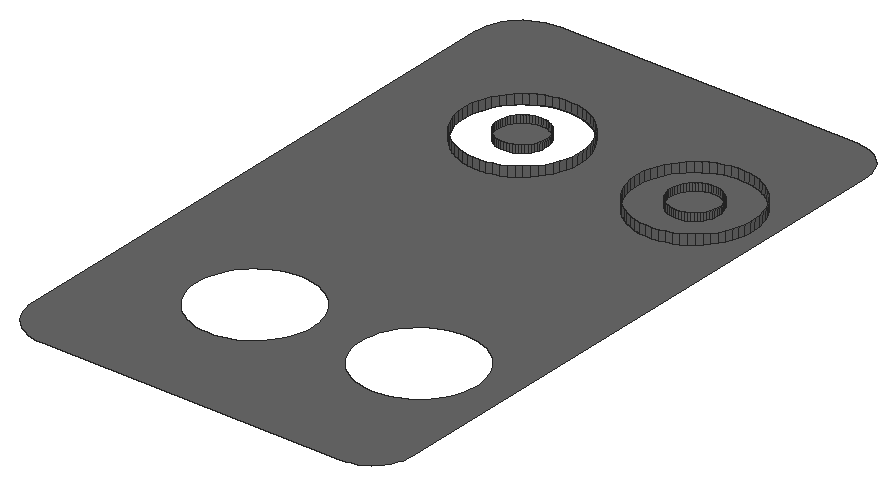
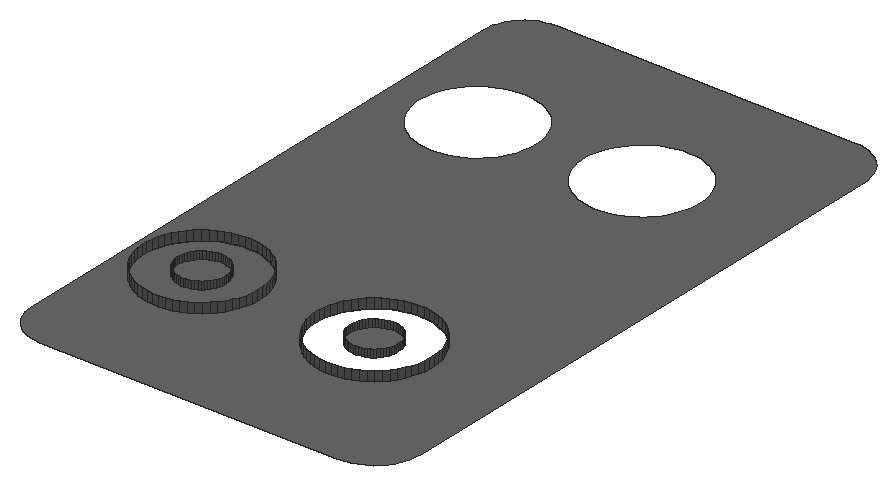
# SketchUp Ruby script. Lengths in inches.
U = 1.inch
M = Sketchup.active_model
def pt(a) = Geom::Point3d.new(a.map { |v| v * U })
def face(e, loops, mat)
  f = e.add_face(loops[0].map { |a| pt(a) })
  loops[1..].each { |l| e.add_face(l.map { |a| pt(a) }).erase! }
  f.material = f.back_material = mat if mat
  f
end
# faces: each face lists its corners as indices into pts; further lists are holes
def faces(e, pts, list, mat = nil) = list.each { |f| face(e, (f[0].is_a?(Array) ? f : [f]).map { |l| l.map { |i| pts[i] } }, mat) }
# xy, xz, yz: faces in a plane at the given z, y or x. An outline is a flat list of corners, or four numbers for a rectangle; further outlines are holes
def ring(l) = l.size == 4 ? [[l[0], l[1]], [l[2], l[1]], [l[2], l[3]], [l[0], l[3]]] : l.each_slice(2).to_a
def flat(e, list, mat, &to3) = list.each { |f| face(e, (f[0].is_a?(Array) ? f : [f]).map { |l| ring(l).map { |u, v| to3.(u, v) } }, mat) }
def xy(e, z, list, mat = nil) = flat(e, list, mat) { |x, y| [x, y, z] }
def xz(e, y, list, mat = nil) = flat(e, list, mat) { |x, z| [x, y, z] }
def yz(e, x, list, mat = nil) = flat(e, list, mat) { |y, z| [x, y, z] }
def lines(e, pts, list) = list.each { |a, b| e.add_line(pt(pts[a]), pt(pts[b])) }
# prism: a flat outline (further loops are holes) pulled along v
def prism(e, loops, v, mat = nil)
  f = face(e, loops, mat); d = Geom::Vector3d.new(v.map { |x| x * U })
  f.pushpull(f.normal.samedirection?(d) ? d.length : -d.length)
end
def box(e, o, s, mat = nil) = prism(e, [[o, [o[0] + s[0], o[1], o[2]], [o[0] + s[0], o[1] + s[1], o[2]], [o[0], o[1] + s[1], o[2]]]], [0, 0, s[2]], mat)
def at(x, y, z, deg = 0) = Geom::Transformation.translation(pt([x, y, z])) * Geom::Transformation.rotation(ORIGIN, Z_AXIS, deg.degrees)
def axes(o, x, y, z) = Geom::Transformation.new([*x, 0, *y, 0, *z, 0, *pt(o).to_a, 1])
def part(name) = M.definitions.add(name)
# library, detail: a bought-in or finely detailed component or shape, given as its bounding box
def library(name, o, s) = part(name).tap { |d| box(d.entities, o, s) }
def detail(e, o, s) = box(e.add_group.entities, o, s)
def put(e, d, t, mat = nil) = e.add_instance(d, t).tap { |i| i.material = mat if mat }
def group(e, t, mat = nil) = e.add_group.tap { |g| g.transformation = t; g.material = mat if mat }.entities
root = M.entities
M.materials.add("[0134_DimGray]").color = [105, 105, 105]
xy(root,118,[[[56.8,138.66,118.35,138.66,119.44,138.73,120.52,138.94,121.55,139.3,122.54,139.78,123.45,140.39,124.27,141.11,124.99,141.9375,125.6,142.85,126.09,143.83,126.44,144.87,126.65,145.94,126.73,147.04,126.73,263.91,126.65,265,126.44,266.08,126.09,267.11,125.6,268.1,124.99,269.01,124.27,269.83,123.45,270.55,122.54,271.16,121.55,271.65,120.52,272,119.44,272.21,118.35,272.28,56.8,272.28,55.54,272.2,54.3,271.96,53.11,271.55,51.98,270.99,50.93,270.29,49.98,269.46,49.15,268.51,48.45,267.47,47.9,266.34,47.49,265.14,47.25,263.91,47.16,262.65,47.16,148.29,47.25,147.04,47.49,145.8,47.9,144.61,48.45,143.48,49.15,142.43,49.98,141.48,50.93,140.65,51.98,139.95,53.11,139.39,54.3,138.99,55.54,138.74],[75.05,157.99,73.8,158.11,72.57,158.36,71.375,158.74,70.22,159.25,69.13,159.87,68.11,160.6,67.17,161.43,66.33,162.36,65.58,163.37,64.94,164.46,64.43,165.6,64.03,166.79,63.76,168.02,63.62,169.27,63.61,170.52,63.74,171.77,63.99,173,64.37,174.2,64.87,175.35,65.49,176.44,66.22,177.46,67.06,178.4,67.99,179.25,69,179.99,70.08,180.63,71.23,181.15,72.42,181.54,73.64,181.8125,74.89,181.95,76.15,181.96,77.4,181.84,78.63,181.59,79.83,181.21,80.98,180.7,82.07,180.08,83.09,179.35,84.03,178.52,84.875,177.59,85.62,176.58,86.26,175.49,86.77,174.35,87.17,173.16,87.44,171.93,87.58,170.68,87.59,169.43,87.46,168.18,87.21,166.95,86.83,165.75,86.33,164.6,85.71,163.51,84.98,162.48,84.14,161.55,83.21,160.7,82.2,159.95,81.12,159.32,79.98,158.8,78.78,158.4,77.56,158.13,76.31,158],[75.05,227.2,73.8,227.32,72.57,227.58,71.375,227.96,70.22,228.46,69.13,229.08,68.11,229.8125,67.17,230.65,66.33,231.57,65.58,232.58,64.94,233.67,64.43,234.8125,64.03,236,63.76,237.23,63.62,238.48,63.61,239.74,63.74,240.99,63.99,242.22,64.37,243.41,64.87,244.5625,65.49,245.66,66.22,246.68,67.06,247.62,67.99,248.46,69,249.21,70.08,249.84,71.23,250.36,72.42,250.76,73.64,251.03,74.89,251.17,76.15,251.18,77.4,251.05,78.63,250.8,79.83,250.42,80.98,249.92,82.07,249.3,83.09,248.5625,84.03,247.73,84.875,246.8,85.62,245.79,86.26,244.71,86.77,243.5625,87.17,242.37,87.44,241.14,87.58,239.9,87.59,238.64,87.46,237.39,87.21,236.16,86.83,234.96,86.33,233.8125,85.71,232.72,84.98,231.7,84.14,230.76,83.21,229.91,82.2,229.17,81.12,228.53,79.98,228.01,78.78,227.62,77.56,227.35,76.31,227.21],[107.89,159.41,106.64,159.53,105.41,159.78,104.21,160.16,103.0625,160.67,101.97,161.29,100.95,162.02,100.01,162.85,99.16,163.78,98.42,164.79,97.78,165.875,97.26,167.02,96.87,168.21,96.6,169.4375,96.46,170.6875,96.45,171.94,96.57,173.19,96.83,174.42,97.21,175.62,97.71,176.77,98.33,177.86,99.0625,178.88,99.9,179.82,100.82,180.67,101.84,181.42,102.92,182.05,104.0625,182.57,105.26,182.97,106.48,183.23,107.73,183.375,108.99,183.38,110.24,183.26,111.47,183.01,112.66,182.625,113.81,182.125,114.91,181.5,115.93,180.77,116.87,179.9375,117.71,179.01,118.46,178,119.09,176.91,119.61,175.77,120.01,174.58,120.28,173.35,120.42,172.1,120.43,170.85,120.3,169.6,120.05,168.37,119.67,167.17,119.17,166.02,118.55,164.93,117.8125,163.91,116.98,162.97,116.05,162.12,115.04,161.375,113.96,160.74,112.8125,160.22,111.62,159.83,110.39,159.56,109.15,159.42],[110.81,227.1,109.56,227.22,108.33,227.47,107.13,227.85,105.98,228.36,104.89,228.98,103.86,229.71,102.93,230.54,102.08,231.47,101.33,232.48,100.7,233.57,100.18,234.71,99.78,235.9,99.51,237.13,99.375,238.38,99.37,239.63,99.49,240.88,99.74,242.11,100.12,243.3125,100.625,244.46,101.25,245.55,101.98,246.58,102.8125,247.51,103.74,248.36,104.75,249.11,105.83,249.74,106.98,250.26,108.17,250.66,109.4,250.93,110.65,251.07,111.9,251.07,113.15,250.95,114.38,250.7,115.58,250.32,116.73,249.81,117.82,249.19,118.84,248.46,119.78,247.63,120.63,246.7,121.375,245.6875,122.01,244.61,122.53,243.46,122.92,242.27,123.19,241.04,123.33,239.79,123.34,238.54,123.22,237.29,122.97,236.06,122.59,234.86,122.08,233.71,121.46,232.62,120.73,231.6,119.9,230.66,118.97,229.8125,117.96,229.07,116.875,228.43,115.73,227.91,114.54,227.52,113.31,227.25,112.0625,227.11]],[110.81,227.1,109.56,227.22,108.33,227.47,107.13,227.85,105.98,228.36,104.89,228.98,103.86,229.71,102.93,230.54,102.08,231.47,101.33,232.48,100.7,233.57,100.18,234.71,99.78,235.9,99.51,237.13,99.375,238.38,99.37,239.63,99.49,240.88,99.74,242.11,100.12,243.3125,100.625,244.46,101.25,245.55,101.98,246.58,102.8125,247.51,103.74,248.36,104.75,249.11,105.83,249.74,106.98,250.26,108.17,250.66,109.4,250.93,110.65,251.07,111.9,251.07,113.15,250.95,114.38,250.7,115.58,250.32,116.73,249.81,117.82,249.19,118.84,248.46,119.78,247.63,120.63,246.7,121.375,245.6875,122.01,244.61,122.53,243.46,122.92,242.27,123.19,241.04,123.33,239.79,123.34,238.54,123.22,237.29,122.97,236.06,122.59,234.86,122.08,233.71,121.46,232.62,120.73,231.6,119.9,230.66,118.97,229.8125,117.96,229.07,116.875,228.43,115.73,227.91,114.54,227.52,113.31,227.25,112.0625,227.11]],"[0134_DimGray]")
xy(root,118.5,[[111.53,234.09,112.05,234.14,112.5625,234.23,113.0625,234.39,113.55,234.59,114,234.85,114.43,235.15,114.83,235.49,115.18,235.87,115.5,236.29,115.77,236.74,115.99,237.21,116.16,237.71,116.28,238.22,116.34,238.74,116.35,239.26,116.31,239.78,116.21,240.3,116.05,240.8,115.85,241.28,115.59,241.74,115.29,242.16,114.95,242.56,114.57,242.92,114.15,243.23,113.7,243.5,113.23,243.72,112.73,243.89,112.22,244.01,111.7,244.07,111.18,244.08,110.66,244.04,110.14,243.9375,109.64,243.78,109.16,243.58,108.7,243.33,108.28,243.03,107.88,242.68,107.52,242.3,107.21,241.88,106.9375,241.43,106.72,240.96,106.55,240.46,106.43,239.95,106.37,239.44,106.36,238.91,106.4,238.39,106.5,237.875,106.66,237.375,106.86,236.89,107.11,236.4375,107.41,236.01,107.76,235.61,108.14,235.26,108.56,234.94,109.01,234.67,109.48,234.45,109.98,234.28,110.49,234.16,111.01,234.1],[75.77,234.19,76.3,234.24,76.81,234.34,77.31,234.49,77.79,234.69,78.25,234.95,78.68,235.25,79.07,235.59,79.43,235.97,79.75,236.39,80.01,236.84,80.24,237.31,80.41,237.81,80.52,238.32,80.59,238.84,80.6,239.36,80.55,239.88,80.45,240.4,80.3,240.9,80.09,241.38,79.84,241.84,79.54,242.27,79.2,242.66,78.8125,243.02,78.4,243.33,77.95,243.6,77.47,243.82,76.98,243.99,76.47,244.11,75.95,244.18,75.43,244.18,74.9,244.14,74.39,244.04,73.89,243.89,73.41,243.68,72.95,243.43,72.52,243.13,72.125,242.78,71.77,242.4,71.45,241.98,71.19,241.53,70.96,241.0625,70.79,240.57,70.68,240.06,70.61,239.54,70.6,239.01,70.65,238.49,70.75,237.98,70.9,237.48,71.11,237,71.36,236.54,71.66,236.11,72,235.71,72.39,235.36,72.8,235.04,73.25,234.77,73.73,234.55,74.22,234.38,74.73,234.26,75.25,234.2]],"[0134_DimGray]")
xz(root,244.18,[[75.43,118.5,75.95,120]],"[0134_DimGray]")
xz(root,251.07,[[110.65,118,111.9,120]],"[0134_DimGray]")
p = [[109.56,227.22,118],[110.81,227.1,118],[110.81,227.1,120],[109.56,227.22,120],[112.0625,227.11,118],[112.0625,227.11,120],
  [113.31,227.25,118],[113.31,227.25,120],[73.8,227.32,118],[75.05,227.2,118],[75.05,227.2,120],[73.8,227.32,120],
  [76.31,227.21,118],[76.31,227.21,120],[77.56,227.35,118],[77.56,227.35,120],[108.33,227.47,118],[108.33,227.47,120],
  [114.54,227.52,118],[114.54,227.52,120],[72.57,227.58,118],[72.57,227.58,120],[78.78,227.62,118],[78.78,227.62,120],
  [107.13,227.85,118],[107.13,227.85,120],[115.73,227.91,118],[115.73,227.91,120],[71.375,227.96,118],[71.375,227.96,120],
  [79.98,228.01,118],[79.98,228.01,120],[105.98,228.36,118],[105.98,228.36,120],[116.875,228.43,118],[116.875,228.43,120],
  [70.22,228.46,118],[70.22,228.46,120],[81.12,228.53,118],[81.12,228.53,120],[104.89,228.98,118],[104.89,228.98,120],
  [117.96,229.07,118],[117.96,229.07,120],[69.13,229.08,118],[69.13,229.08,120],[82.2,229.17,118],[82.2,229.17,120],
  [103.86,229.71,118],[103.86,229.71,120],[68.11,229.8125,118],[68.11,229.8125,120],[118.97,229.8125,118],[118.97,229.8125,120],
  [83.21,229.91,118],[83.21,229.91,120],[102.93,230.54,118],[102.93,230.54,120],[67.17,230.65,118],[67.17,230.65,120],
  [119.9,230.66,118],[119.9,230.66,120],[84.14,230.76,118],[84.14,230.76,120],[102.08,231.47,118],[102.08,231.47,120],
  [66.33,231.57,118],[66.33,231.57,120],[120.73,231.6,118],[120.73,231.6,120],[84.98,231.7,118],[84.98,231.7,120],
  [101.33,232.48,118],[101.33,232.48,120],[65.58,232.58,118],[65.58,232.58,120],[121.46,232.62,118],[121.46,232.62,120],
  [85.71,232.72,118],[85.71,232.72,120],[100.7,233.57,118],[100.7,233.57,120],[64.94,233.67,118],[64.94,233.67,120],
  [122.08,233.71,118],[122.08,233.71,120],[86.33,233.8125,118],[86.33,233.8125,120],[100.18,234.71,118],[100.18,234.71,120],
  [64.43,234.8125,118],[64.43,234.8125,120],[122.59,234.86,118],[122.59,234.86,120],[86.83,234.96,118],[86.83,234.96,120],
  [99.78,235.9,118],[99.78,235.9,120],[64.03,236,118],[64.03,236,120],[122.97,236.06,118],[122.97,236.06,120],
  [87.21,236.16,118],[87.21,236.16,120],[99.51,237.13,118],[99.51,237.13,120],[63.76,237.23,118],[63.76,237.23,120],
  [123.22,237.29,118],[123.22,237.29,120],[87.46,237.39,118],[87.46,237.39,120],[99.375,238.38,118],[99.375,238.38,120],
  [63.62,238.48,118],[63.62,238.48,120],[123.34,238.54,118],[123.34,238.54,120],[87.59,238.64,118],[87.59,238.64,120],
  [99.37,239.63,118],[99.37,239.63,120],[63.61,239.74,118],[63.61,239.74,120],[123.33,239.79,118],[123.33,239.79,120],
  [87.58,239.9,118],[87.58,239.9,120],[99.49,240.88,118],[99.49,240.88,120],[63.74,240.99,118],[63.74,240.99,120],
  [123.19,241.04,118],[123.19,241.04,120],[87.44,241.14,118],[87.44,241.14,120],[99.74,242.11,118],[99.74,242.11,120],
  [63.99,242.22,118],[63.99,242.22,120],[122.92,242.27,118],[122.92,242.27,120],[87.17,242.37,118],[87.17,242.37,120],
  [100.12,243.3125,118],[100.12,243.3125,120],[64.37,243.41,118],[64.37,243.41,120],[122.53,243.46,118],[122.53,243.46,120],
  [86.77,243.5625,118],[86.77,243.5625,120],[100.625,244.46,118],[100.625,244.46,120],[64.87,244.5625,118],[64.87,244.5625,120],
  [122.01,244.61,118],[122.01,244.61,120],[86.26,244.71,118],[86.26,244.71,120],[101.25,245.55,118],[101.25,245.55,120],
  [65.49,245.66,118],[65.49,245.66,120],[121.375,245.6875,118],[121.375,245.6875,120],[85.62,245.79,118],[85.62,245.79,120],
  [101.98,246.58,118],[101.98,246.58,120],[66.22,246.68,118],[66.22,246.68,120],[120.63,246.7,118],[120.63,246.7,120],
  [84.875,246.8,118],[84.875,246.8,120],[102.8125,247.51,118],[102.8125,247.51,120],[67.06,247.62,118],[67.06,247.62,120],
  [119.78,247.63,118],[119.78,247.63,120],[84.03,247.73,118],[84.03,247.73,120],[103.74,248.36,118],[103.74,248.36,120],
  [67.99,248.46,118],[67.99,248.46,120],[118.84,248.46,118],[118.84,248.46,120],[83.09,248.5625,118],[83.09,248.5625,120],
  [104.75,249.11,118],[104.75,249.11,120],[69,249.21,118],[69,249.21,120],[117.82,249.19,118],[117.82,249.19,120],
  [82.07,249.3,118],[82.07,249.3,120],[105.83,249.74,118],[105.83,249.74,120],[70.08,249.84,118],[70.08,249.84,120],
  [116.73,249.81,118],[116.73,249.81,120],[80.98,249.92,118],[80.98,249.92,120],[106.98,250.26,118],[106.98,250.26,120],
  [71.23,250.36,118],[71.23,250.36,120],[115.58,250.32,118],[115.58,250.32,120],[79.83,250.42,118],[79.83,250.42,120],
  [108.17,250.66,118],[108.17,250.66,120],[114.38,250.7,118],[114.38,250.7,120],[72.42,250.76,118],[72.42,250.76,120],
  [78.63,250.8,118],[78.63,250.8,120],[109.4,250.93,118],[109.4,250.93,120],[113.15,250.95,118],[113.15,250.95,120],
  [73.64,251.03,118],[73.64,251.03,120],[77.4,251.05,118],[77.4,251.05,120],[110.65,251.07,118],[110.65,251.07,120],
  [74.89,251.17,118],[74.89,251.17,120],[111.9,251.07,118],[111.9,251.07,120],[76.15,251.18,118],[76.15,251.18,120],
  [110.49,234.16,120],[111.01,234.1,120],[111.01,234.1,118.5],[110.49,234.16,118.5],[111.53,234.09,120],[111.53,234.09,118.5],
  [112.05,234.14,120],[112.05,234.14,118.5],[112.5625,234.23,120],[112.5625,234.23,118.5],[74.73,234.26,120],[75.25,234.2,120],
  [75.25,234.2,118.5],[74.73,234.26,118.5],[75.77,234.19,120],[75.77,234.19,118.5],[76.3,234.24,120],[76.3,234.24,118.5],
  [76.81,234.34,120],[76.81,234.34,118.5],[109.98,234.28,120],[109.98,234.28,118.5],[113.0625,234.39,120],[113.0625,234.39,118.5],
  [74.22,234.38,120],[74.22,234.38,118.5],[77.31,234.49,120],[77.31,234.49,118.5],[109.48,234.45,120],[109.48,234.45,118.5],
  [73.73,234.55,120],[73.73,234.55,118.5],[113.55,234.59,120],[113.55,234.59,118.5],[77.79,234.69,120],[77.79,234.69,118.5],
  [109.01,234.67,120],[109.01,234.67,118.5],[73.25,234.77,120],[73.25,234.77,118.5],[114,234.85,120],[114,234.85,118.5],
  [78.25,234.95,120],[78.25,234.95,118.5],[108.56,234.94,120],[108.56,234.94,118.5],[72.8,235.04,120],[72.8,235.04,118.5],
  [114.43,235.15,120],[114.43,235.15,118.5],[78.68,235.25,120],[78.68,235.25,118.5],[108.14,235.26,120],[108.14,235.26,118.5],
  [72.39,235.36,120],[72.39,235.36,118.5],[114.83,235.49,120],[114.83,235.49,118.5],[79.07,235.59,120],[79.07,235.59,118.5],
  [107.76,235.61,120],[107.76,235.61,118.5],[72,235.71,120],[72,235.71,118.5],[115.18,235.87,120],[115.18,235.87,118.5],
  [79.43,235.97,120],[79.43,235.97,118.5],[107.41,236.01,120],[107.41,236.01,118.5],[71.66,236.11,120],[71.66,236.11,118.5],
  [115.5,236.29,120],[115.5,236.29,118.5],[79.75,236.39,120],[79.75,236.39,118.5],[107.11,236.4375,120],[107.11,236.4375,118.5],
  [71.36,236.54,120],[71.36,236.54,118.5],[115.77,236.74,120],[115.77,236.74,118.5],[80.01,236.84,120],[80.01,236.84,118.5],
  [106.86,236.89,120],[106.86,236.89,118.5],[71.11,237,120],[71.11,237,118.5],[115.99,237.21,120],[115.99,237.21,118.5],
  [80.24,237.31,120],[80.24,237.31,118.5],[106.66,237.375,120],[106.66,237.375,118.5],[70.9,237.48,120],[70.9,237.48,118.5],
  [116.16,237.71,120],[116.16,237.71,118.5],[80.41,237.81,120],[80.41,237.81,118.5],[106.5,237.875,120],[106.5,237.875,118.5],
  [70.75,237.98,120],[70.75,237.98,118.5],[116.28,238.22,120],[116.28,238.22,118.5],[80.52,238.32,120],[80.52,238.32,118.5],
  [106.4,238.39,120],[106.4,238.39,118.5],[70.65,238.49,120],[70.65,238.49,118.5],[116.34,238.74,120],[116.34,238.74,118.5],
  [80.59,238.84,120],[80.59,238.84,118.5],[106.36,238.91,120],[106.36,238.91,118.5],[70.6,239.01,120],[70.6,239.01,118.5],
  [116.35,239.26,120],[116.35,239.26,118.5],[80.6,239.36,120],[80.6,239.36,118.5],[106.37,239.44,120],[106.37,239.44,118.5],
  [70.61,239.54,120],[70.61,239.54,118.5],[116.31,239.78,120],[116.31,239.78,118.5],[80.55,239.88,120],[80.55,239.88,118.5],
  [106.43,239.95,120],[106.43,239.95,118.5],[70.68,240.06,120],[70.68,240.06,118.5],[116.21,240.3,120],[116.21,240.3,118.5],
  [80.45,240.4,120],[80.45,240.4,118.5],[106.55,240.46,120],[106.55,240.46,118.5],[70.79,240.57,120],[70.79,240.57,118.5],
  [116.05,240.8,120],[116.05,240.8,118.5],[80.3,240.9,120],[80.3,240.9,118.5],[106.72,240.96,120],[106.72,240.96,118.5],
  [70.96,241.0625,120],[70.96,241.0625,118.5],[115.85,241.28,120],[115.85,241.28,118.5],[80.09,241.38,120],[80.09,241.38,118.5],
  [106.9375,241.43,120],[106.9375,241.43,118.5],[71.19,241.53,120],[71.19,241.53,118.5],[115.59,241.74,120],[115.59,241.74,118.5],
  [79.84,241.84,120],[79.84,241.84,118.5],[107.21,241.88,120],[107.21,241.88,118.5],[71.45,241.98,120],[71.45,241.98,118.5],
  [115.29,242.16,120],[115.29,242.16,118.5],[79.54,242.27,120],[79.54,242.27,118.5],[107.52,242.3,120],[107.52,242.3,118.5],
  [71.77,242.4,120],[71.77,242.4,118.5],[114.95,242.56,120],[114.95,242.56,118.5],[79.2,242.66,120],[79.2,242.66,118.5],
  [107.88,242.68,120],[107.88,242.68,118.5],[72.125,242.78,120],[72.125,242.78,118.5],[114.57,242.92,120],[114.57,242.92,118.5],
  [78.8125,243.02,120],[78.8125,243.02,118.5],[108.28,243.03,120],[108.28,243.03,118.5],[72.52,243.13,120],[72.52,243.13,118.5],
  [114.15,243.23,120],[114.15,243.23,118.5],[78.4,243.33,120],[78.4,243.33,118.5],[108.7,243.33,120],[108.7,243.33,118.5],
  [72.95,243.43,120],[72.95,243.43,118.5],[113.7,243.5,120],[113.7,243.5,118.5],[77.95,243.6,120],[77.95,243.6,118.5],
  [109.16,243.58,120],[109.16,243.58,118.5],[73.41,243.68,120],[73.41,243.68,118.5],[113.23,243.72,120],[113.23,243.72,118.5],
  [77.47,243.82,120],[77.47,243.82,118.5],[109.64,243.78,120],[109.64,243.78,118.5],[73.89,243.89,120],[73.89,243.89,118.5],
  [112.73,243.89,120],[112.73,243.89,118.5],[76.98,243.99,120],[76.98,243.99,118.5],[110.14,243.9375,120],[110.14,243.9375,118.5],
  [74.39,244.04,120],[74.39,244.04,118.5],[110.66,244.04,120],[110.66,244.04,118.5],[112.22,244.01,120],[112.22,244.01,118.5],
  [74.9,244.14,120],[74.9,244.14,118.5],[76.47,244.11,120],[76.47,244.11,118.5],[111.18,244.08,120],[111.18,244.08,118.5],
  [111.7,244.07,120],[111.7,244.07,118.5],[75.43,244.18,120],[75.43,244.18,118.5],[75.95,244.18,120],[75.95,244.18,118.5]]
faces(root,p,[[0,1,2,3],[1,4,5,2],[4,6,7,5],[8,9,10,11],[9,12,13,10],[12,14,15,13],[16,0,3,17],[6,18,19,7],
  [20,8,11,21],[14,22,23,15],[24,16,17,25],[18,26,27,19],[28,20,21,29],[22,30,31,23],[32,24,25,33],[26,34,35,27],
  [36,28,29,37],[30,38,39,31],[40,32,33,41],[34,42,43,35],[44,36,37,45],[38,46,47,39],[48,40,41,49],[50,44,45,51],
  [42,52,53,43],[46,54,55,47],[56,48,49,57],[58,50,51,59],[52,60,61,53],[54,62,63,55],[64,56,57,65],[66,58,59,67],
  [60,68,69,61],[62,70,71,63],[72,64,65,73],[74,66,67,75],[68,76,77,69],[70,78,79,71],[80,72,73,81],[82,74,75,83],
  [76,84,85,77],[78,86,87,79],[88,80,81,89],[90,82,83,91],[84,92,93,85],[86,94,95,87],[96,88,89,97],[98,90,91,99],
  [92,100,101,93],[94,102,103,95],[104,96,97,105],[106,98,99,107],[100,108,109,101],[102,110,111,103],[112,104,105,113],[114,106,107,115],
  [108,116,117,109],[110,118,119,111],[120,112,113,121],[122,114,115,123],[116,124,125,117],[118,126,127,119],[128,120,121,129],[130,122,123,131],
  [124,132,133,125],[126,134,135,127],[136,128,129,137],[138,130,131,139],[132,140,141,133],[134,142,143,135],[144,136,137,145],[146,138,139,147],
  [140,148,149,141],[142,150,151,143],[152,144,145,153],[154,146,147,155],[148,156,157,149],[150,158,159,151],[160,152,153,161],[162,154,155,163],
  [156,164,165,157],[158,166,167,159],[168,160,161,169],[170,162,163,171],[164,172,173,165],[166,174,175,167],[176,168,169,177],[178,170,171,179],
  [172,180,181,173],[174,182,183,175],[184,176,177,185],[186,178,179,187],[180,188,189,181],[182,190,191,183],[192,184,185,193],[194,186,187,195],
  [188,196,197,189],[190,198,199,191],[200,192,193,201],[202,194,195,203],[196,204,205,197],[198,206,207,199],[208,200,201,209],[210,202,203,211],
  [204,212,213,205],[206,214,215,207],[216,208,209,217],[212,218,219,213],[220,210,211,221],[214,222,223,215],[224,216,217,225],[218,226,227,219],
  [228,220,221,229],[222,230,231,223],[232,224,225,233],[234,228,229,235],[226,236,237,227],[230,238,239,231],[238,234,235,239],[240,241,242,243],
  [241,244,245,242],[244,246,247,245],[246,248,249,247],[250,251,252,253],[251,254,255,252],[254,256,257,255],[256,258,259,257],[260,240,243,261],
  [248,262,263,249],[264,250,253,265],[258,266,267,259],[268,260,261,269],[270,264,265,271],[262,272,273,263],[266,274,275,267],[276,268,269,277],
  [278,270,271,279],[272,280,281,273],[274,282,283,275],[284,276,277,285],[286,278,279,287],[280,288,289,281],[282,290,291,283],[292,284,285,293],
  [294,286,287,295],[288,296,297,289],[290,298,299,291],[300,292,293,301],[302,294,295,303],[296,304,305,297],[298,306,307,299],[308,300,301,309],
  [310,302,303,311],[304,312,313,305],[306,314,315,307],[316,308,309,317],[318,310,311,319],[312,320,321,313],[314,322,323,315],[324,316,317,325],
  [326,318,319,327],[320,328,329,321],[322,330,331,323],[332,324,325,333],[334,326,327,335],[328,336,337,329],[330,338,339,331],[340,332,333,341],
  [342,334,335,343],[336,344,345,337],[338,346,347,339],[348,340,341,349],[350,342,343,351],[344,352,353,345],[346,354,355,347],[356,348,349,357],
  [358,350,351,359],[352,360,361,353],[354,362,363,355],[364,356,357,365],[366,358,359,367],[360,368,369,361],[362,370,371,363],[372,364,365,373],
  [374,366,367,375],[368,376,377,369],[370,378,379,371],[380,372,373,381],[382,374,375,383],[376,384,385,377],[378,386,387,379],[388,380,381,389],
  [390,382,383,391],[384,392,393,385],[386,394,395,387],[396,388,389,397],[398,390,391,399],[392,400,401,393],[394,402,403,395],[404,396,397,405],
  [406,398,399,407],[400,408,409,401],[402,410,411,403],[412,404,405,413],[414,406,407,415],[408,416,417,409],[410,418,419,411],[420,412,413,421],
  [422,414,415,423],[416,424,425,417],[418,426,427,419],[428,420,421,429],[430,422,423,431],[424,432,433,425],[426,434,435,427],[436,428,429,437],
  [438,430,431,439],[432,440,441,433],[434,442,443,435],[444,436,437,445],[446,438,439,447],[440,448,449,441],[442,450,451,443],[452,444,445,453],
  [454,446,447,455],[448,456,457,449],[450,458,459,451],[460,452,453,461],[462,454,455,463],[464,460,461,465],[456,466,467,457],[468,462,463,469],
  [458,470,471,459],[472,464,465,473],[466,474,475,467],[476,468,469,477],[470,478,479,471],[474,472,473,475]],"[0134_DimGray]")
